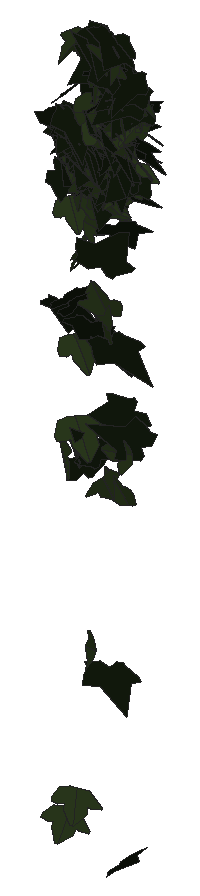
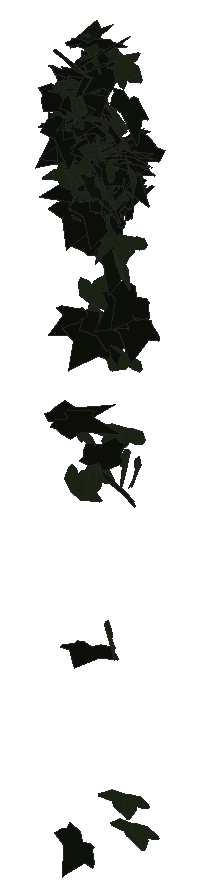
# SketchUp Ruby script. Lengths in inches.
U = 1.inch
M = Sketchup.active_model
def pt(a) = Geom::Point3d.new(a.map { |v| v * U })
def face(e, loops, mat)
  f = e.add_face(loops[0].map { |a| pt(a) })
  loops[1..].each { |l| e.add_face(l.map { |a| pt(a) }).erase! }
  f.material = f.back_material = mat if mat
  f
end
# faces: each face lists its corners as indices into pts; further lists are holes
def faces(e, pts, list, mat = nil) = list.each { |f| face(e, (f[0].is_a?(Array) ? f : [f]).map { |l| l.map { |i| pts[i] } }, mat) }
# xy, xz, yz: faces in a plane at the given z, y or x. An outline is a flat list of corners, or four numbers for a rectangle; further outlines are holes
def ring(l) = l.size == 4 ? [[l[0], l[1]], [l[2], l[1]], [l[2], l[3]], [l[0], l[3]]] : l.each_slice(2).to_a
def flat(e, list, mat, &to3) = list.each { |f| face(e, (f[0].is_a?(Array) ? f : [f]).map { |l| ring(l).map { |u, v| to3.(u, v) } }, mat) }
def xy(e, z, list, mat = nil) = flat(e, list, mat) { |x, y| [x, y, z] }
def xz(e, y, list, mat = nil) = flat(e, list, mat) { |x, z| [x, y, z] }
def yz(e, x, list, mat = nil) = flat(e, list, mat) { |y, z| [x, y, z] }
def lines(e, pts, list) = list.each { |a, b| e.add_line(pt(pts[a]), pt(pts[b])) }
# prism: a flat outline (further loops are holes) pulled along v
def prism(e, loops, v, mat = nil)
  f = face(e, loops, mat); d = Geom::Vector3d.new(v.map { |x| x * U })
  f.pushpull(f.normal.samedirection?(d) ? d.length : -d.length)
end
def box(e, o, s, mat = nil) = prism(e, [[o, [o[0] + s[0], o[1], o[2]], [o[0] + s[0], o[1] + s[1], o[2]], [o[0], o[1] + s[1], o[2]]]], [0, 0, s[2]], mat)
def at(x, y, z, deg = 0) = Geom::Transformation.translation(pt([x, y, z])) * Geom::Transformation.rotation(ORIGIN, Z_AXIS, deg.degrees)
def axes(o, x, y, z) = Geom::Transformation.new([*x, 0, *y, 0, *z, 0, *pt(o).to_a, 1])
def part(name) = M.definitions.add(name)
# library, detail: a bought-in or finely detailed component or shape, given as its bounding box
def library(name, o, s) = part(name).tap { |d| box(d.entities, o, s) }
def detail(e, o, s) = box(e.add_group.entities, o, s)
def put(e, d, t, mat = nil) = e.add_instance(d, t).tap { |i| i.material = mat if mat }
def group(e, t, mat = nil) = e.add_group.tap { |g| g.transformation = t; g.material = mat if mat }.entities
root = M.entities
M.materials.add("1026 AP 7946 SUNNY SIDE UP").color = [254, 231, 186]
M.materials.add("efeu1").color = [18, 25, 13]
M.materials.add("efeu2").color = [43, 57, 29]
c1 = part("ivyleaf_9")
p = [[1.54,2.16,1.25],[1.36,2.04,1.19],[-0.21,0.99,0.68],[-0.71,1.11,0.82],[-0.85,0.86,0.67],[-0.8,0.17,0.21],
  [-0.9,-0.01,0.1],[-0.67,-0.16,-0.02],[-0.08,-0.08,-0.05],[-0.03,-0.6,-0.4],[0.65,-0.88,-0.66],[0.83,-0.6,-0.49],
  [1.29,-0.42,-0.43],[1.8125,-0.07,-0.26],[1.21,0.44,0.15]]
faces(c1.entities,p,[[0,1,2,3,4,5,6,7,8,9,10,11,12,13,14]],"efeu1")
c2 = part("ivyleaf_10")
p = [[0,0.5,-0.03],[-0.0625,2.02,-0.43],[-0.19,2.01,-0.46],[-0.54,1.05,-0.29],[-0.52,0.625,-0.18],[-0.83,0.76,-0.28],
  [-1.16,0.64,-0.33],[-1.15,0.33,-0.24],[-0.77,-0.39,0.02],[-0.3,-0.51,0.16],[0.04,-0.48,0.23],[-0.02,2.01,-0.4375],
  [-0.06,2.01,-0.43],[0.04,-0.49,0.23],[0.67,-0.49,0.14],[1.38,0.36,-0.2],[1.375,0.51,-0.24],[0.81,0.65,-0.19],
  [0.62,0.59,-0.15],[0.6,1.09,-0.28],[0.5,1.23,-0.31]]
faces(c2.entities,p,[[0,1,2,3,4,5,6,7,8,9,10],[11,12,0,13,14,15,16,17,18,19,20]],"efeu2")
put(root,c1,axes([114.61,212.93,265.6875],[-0.05333,0.19687,-0.14249],[-0.05578,-0.14334,-0.20046],[-0.37521,-0.00667,0.05006]),"1026 AP 7946 SUNNY SIDE UP")
put(root,c2,axes([114.4,212.68,259.63],[-0.11326,0.21899,-0.07805],[0.0251,-0.07577,-0.23779],[-0.36414,-0.07333,0.00789]),"1026 AP 7946 SUNNY SIDE UP")
put(root,c1,axes([114.48,212.61,262.48],[0.29734,0.09526,-0.11901],[-0.13937,-0.07983,-0.21675],[-0.19058,0.20702,-0.02717]),"1026 AP 7946 SUNNY SIDE UP")
put(root,c2,axes([114.38,212.92,264.26],[0.24145,0.1835,0.03806],[0.03802,0.02658,-0.24634],[-0.29154,0.15544,-0.00061]),"1026 AP 7946 SUNNY SIDE UP")
put(root,c1,axes([114.33,212.96,265.49],[0.20834,-0.19966,-0.05353],[-0.06361,0.03404,-0.2462],[0.31765,0.13777,-0.01419]),"1026 AP 7946 SUNNY SIDE UP")
put(root,c1,axes([114.4,212.9,264.9375],[-0.05589,-0.1113,0.21897],[-0.01073,-0.21494,-0.11804],[0.37799,-0.02256,0.02903]),"1026 AP 7946 SUNNY SIDE UP")
put(root,c2,axes([114.48,212.67,252.5],[0.38235,0.02143,-0.02276],[-0.03132,-0.02579,-0.25042],[-0.03706,0.24281,-0.02314]),"1026 AP 7946 SUNNY SIDE UP")
put(root,c2,axes([114.51,212.85,265.91],[0.15682,-0.22679,-0.00735],[0.02996,0.01473,-0.25401],[0.35547,0.09881,0.02465]),"1026 AP 7946 SUNNY SIDE UP")
put(root,c1,axes([114.4,212.53,265.07],[0.19369,-0.10602,-0.21035],[-0.11166,0.20211,-0.15151],[0.34322,0.12558,0.06942]),"1026 AP 7946 SUNNY SIDE UP")
put(root,c2,axes([114.41,212.9,265.57],[-0.23643,0.11477,-0.15666],[0.1408,-0.12933,-0.19171],[-0.26535,-0.17089,0.03785]),"1026 AP 7946 SUNNY SIDE UP")
put(root,c1,axes([114.32,212.95,265.11],[0.05251,-0.03831,-0.24539],[0.35496,-0.07926,0.04532],[-0.13288,-0.22686,0.02408]),"1026 AP 7946 SUNNY SIDE UP")
put(root,c1,axes([114.56,212.96,265.89],[-0.22943,-0.19387,0.04254],[-0.02691,-0.04013,-0.24998],[0.31089,-0.14655,0.00976]),"1026 AP 7946 SUNNY SIDE UP")
put(root,c1,axes([114.67,212.5625,266.77],[-0.03368,0.24703,0.04677],[-0.00032,0.04414,-0.25516],[-0.39454,-0.02112,-0.00379]),"1026 AP 7946 SUNNY SIDE UP")
put(root,c1,axes([114.38,212.9375,265.44],[0.05893,-0.23241,0.06215],[0.02788,-0.05956,-0.24274],[0.37706,0.04073,0.00823]),"1026 AP 7946 SUNNY SIDE UP")
put(root,c1,axes([114.52,212.97,265.73],[-0.26587,-0.16572,-0.06851],[0.10124,0.02747,-0.24243],[0.26131,-0.17926,0.02422]),"1026 AP 7946 SUNNY SIDE UP")
put(root,c1,axes([114.57,212.93,266],[-0.32539,-0.13596,-0.02618],[0.09505,-0.04918,-0.24373],[0.19538,-0.20251,0.07498]),"1026 AP 7946 SUNNY SIDE UP")
put(root,c2,axes([114.57,212.86,267.61],[-0.01298,-0.17717,0.19164],[0.02965,-0.18704,-0.18277],[0.404,0.00804,0.01957]),"1026 AP 7946 SUNNY SIDE UP")
put(root,c2,axes([114.62,212.98,265.69],[-0.04034,-0.24068,0.0225],[-0.00023,-0.02332,-0.24948],[0.38021,-0.02555,0.00224]),"1026 AP 7946 SUNNY SIDE UP")
put(root,c2,axes([114.63,212.68,259.76],[-0.18763,0.19887,0.07935],[-0.0833,0.05653,-0.23806],[-0.32418,-0.12963,0.01524]),"1026 AP 7946 SUNNY SIDE UP")
put(root,c1,axes([114.26,212.67,265.8125],[0.08907,0.00515,0.27764],[0.41543,-0.05551,-0.05645],[0.0838,0.26971,-0.01527]),"1026 AP 7946 SUNNY SIDE UP")
put(root,c1,axes([114.58,212.9375,265.39],[0.2485,-0.09589,-0.16561],[-0.232,0.0645,-0.18933],[0.17992,0.2156,-0.01539]),"1026 AP 7946 SUNNY SIDE UP")
put(root,c2,axes([114.57,212.83,265.39],[-0.13838,0.1416,-0.1832],[0.06251,-0.17902,-0.16742],[-0.35294,-0.08723,0.04218]),"1026 AP 7946 SUNNY SIDE UP")
put(root,c1,axes([114.65,212.93,265.84],[-0.29389,-0.15418,-0.05522],[0.11125,-0.00451,-0.24481],[0.23081,-0.19415,0.04769]),"1026 AP 7946 SUNNY SIDE UP")
put(root,c1,axes([114.76,212.8,259.25],[-0.30001,0.16468,-0.05193],[-0.04194,0.04746,0.25926],[0.26798,0.1918,-0.01756]),"1026 AP 7946 SUNNY SIDE UP")
put(root,c2,axes([114.68,212.7,265.36],[0.34307,-0.10812,0.00827],[0.0109,-0.00548,-0.25088],[0.17021,0.21828,-0.00061]),"1026 AP 7946 SUNNY SIDE UP")
put(root,c1,axes([114.93,212.875,266.33],[-0.01864,0.08351,0.28829],[-0.1234,0.26837,-0.0845],[-0.44157,-0.07852,0.01144]),"1026 AP 7946 SUNNY SIDE UP")
put(root,c2,axes([114.74,212.74,263.66],[0.11866,-0.23815,0.02219],[-0.00014,-0.02403,-0.2574],[0.3762,0.07511,-0.00709]),"1026 AP 7946 SUNNY SIDE UP")
put(root,c1,axes([114.6875,212.38,262.79],[0.15853,0.20494,0.11603],[0.08576,0.09736,-0.23466],[-0.35667,0.1145,-0.00485]),"1026 AP 7946 SUNNY SIDE UP")
put(root,c1,axes([114.64,212.81,265.91],[-0.03721,-0.25365,0.0092],[-0.00123,-0.01034,-0.2625],[0.39917,-0.02367,0.00005]),"1026 AP 7946 SUNNY SIDE UP")
put(root,c1,axes([114.63,212.73,266.125],[-0.03918,-0.25802,-0.01343],[0.01169,0.01091,-0.2669],[0.40595,-0.02522,0.00639]),"1026 AP 7946 SUNNY SIDE UP")
put(root,c1,axes([114.51,212.75,265.2],[0.08159,-0.14421,0.1985],[0.18514,-0.15764,-0.15448],[0.33125,0.12363,0.03745]),"1026 AP 7946 SUNNY SIDE UP")
put(root,c2,axes([114.7,212.63,252.99],[0.3606,0.08865,0.00222],[0.01499,-0.0201,-0.25238],[-0.13862,0.22845,-0.02152]),"1026 AP 7946 SUNNY SIDE UP")
put(root,c2,axes([114.89,212.9,264.64],[-0.13289,0.18179,-0.14206],[-0.07009,0.13219,0.20689],[0.35287,0.09472,-0.0124]),"1026 AP 7946 SUNNY SIDE UP")
put(root,c2,axes([114.78,212.74,264.92],[0.0278,-0.23922,0.07096],[0.08375,-0.06516,-0.24284],[0.38298,0.03161,0.04795]),"1026 AP 7946 SUNNY SIDE UP")
put(root,c2,axes([114.85,212.97,265.15],[-0.26828,-0.16192,0.05873],[0.01197,-0.08862,-0.23265],[0.27014,-0.15688,0.06863]),"1026 AP 7946 SUNNY SIDE UP")
put(root,c1,axes([114.48,212.72,265.46],[0.18973,-0.0468,0.21691],[0.3205,-0.05508,-0.13311],[0.11215,0.23658,0.01344]),"1026 AP 7946 SUNNY SIDE UP")
put(root,c1,axes([114.73,212.49,262.6],[0.17535,0.16565,0.16747],[0.15173,0.12979,-0.20487],[-0.33077,0.14735,-0.0052]),"1026 AP 7946 SUNNY SIDE UP")
put(root,c2,axes([114.83,212.8125,266.27],[-0.3042,0.1507,-0.04565],[0.01363,-0.06128,-0.24921],[-0.247,-0.18898,0.04247]),"1026 AP 7946 SUNNY SIDE UP")
put(root,c1,axes([114.96,212.83,264.88],[-0.05574,0.23506,-0.05008],[0.01517,-0.04906,-0.24517],[-0.37755,-0.03668,-0.00246]),"1026 AP 7946 SUNNY SIDE UP")
put(root,c2,axes([114.87,212.81,264.09],[-0.03218,0.1479,0.19779],[-0.07189,0.186,-0.15222],[-0.37317,-0.04859,0.01227]),"1026 AP 7946 SUNNY SIDE UP")
put(root,c2,axes([114.89,212.9,265.23],[-0.38207,0.01484,-0.00804],[0.00996,-0.02498,-0.24966],[-0.02447,-0.24183,0.02386]),"1026 AP 7946 SUNNY SIDE UP")
put(root,c1,axes([114.6875,212.79,266.02],[0.09518,-0.22147,-0.1124],[0.01517,0.1131,-0.23304],[0.38704,0.05003,0.03678]),"1026 AP 7946 SUNNY SIDE UP")
put(root,c2,axes([114.875,213.02,265.18],[0.2676,-0.17225,-0.00356],[-0.02,-0.00909,-0.249],[0.27014,0.16996,-0.0149]),"1026 AP 7946 SUNNY SIDE UP")
put(root,c2,axes([114.68,212.6875,261.77],[0.33154,0.05044,0.11661],[0.18183,-0.00137,-0.22185],[-0.06887,0.23917,-0.0244]),"1026 AP 7946 SUNNY SIDE UP")
put(root,c1,axes([114.71,212.96,265.08],[0.28332,-0.1529,-0.05402],[-0.08159,0.01829,-0.24254],[0.24026,0.18652,-0.01866]),"1026 AP 7946 SUNNY SIDE UP")
put(root,c2,axes([114.85,212.8125,265.87],[-0.2475,0.16871,-0.08167],[0.02355,-0.09318,-0.23267],[-0.29281,-0.1501,0.05032]),"1026 AP 7946 SUNNY SIDE UP")
put(root,c1,axes([114.95,212.61,263.55],[0.03202,0.21052,0.12117],[0.0253,0.11539,-0.21717],[-0.37743,0.0256,-0.00428]),"1026 AP 7946 SUNNY SIDE UP")
put(root,c2,axes([114.97,212.95,265.19],[-0.14866,0.19543,-0.11407],[-0.06012,0.1056,0.22402],[0.34891,0.10146,-0.01]),"1026 AP 7946 SUNNY SIDE UP")
put(root,c1,axes([114.93,212.94,265.96],[0.23203,0.1536,-0.13166],[-0.12227,-0.10339,-0.21961],[-0.29038,0.16627,-0.01274]),"1026 AP 7946 SUNNY SIDE UP")
put(root,c1,axes([115.07,213.09,265.3],[-0.20652,0.19986,-0.04085],[0.01727,-0.04151,-0.24623],[-0.32027,-0.13111,0.01306]),"1026 AP 7946 SUNNY SIDE UP")
put(root,c2,axes([114.93,212.94,266.05],[0.02504,-0.24775,0.0172],[0.00001,-0.01814,-0.25586],[0.3906,0.01588,-0.0011]),"1026 AP 7946 SUNNY SIDE UP")
put(root,c2,axes([114.76,212.62,260.21],[0.334,0.18375,0.07203],[0.10084,0.03092,-0.28857],[-0.29161,0.22115,-0.01729]),"1026 AP 7946 SUNNY SIDE UP")
put(root,c1,axes([114.87,212.87,265.4],[-0.18611,-0.19906,0.08068],[0.03078,-0.10042,-0.22974],[0.3356,-0.10118,0.06581]),"1026 AP 7946 SUNNY SIDE UP")
put(root,c2,axes([114.89,212.96,265.98],[0.10266,0.23432,0.02189],[-0.04252,0.02802,-0.24804],[-0.36732,0.06225,0.03483]),"1026 AP 7946 SUNNY SIDE UP")
put(root,c2,axes([115.02,212.8,266.08],[-0.38502,-0.02737,0.04223],[-0.05837,-0.03546,-0.25206],[0.0513,-0.24575,0.03018]),"1026 AP 7946 SUNNY SIDE UP")
put(root,c1,axes([114.96,212.93,264.72],[0.21896,0.19792,-0.02089],[-0.02267,-0.01603,-0.24938],[-0.3122,0.13997,0.00345]),"1026 AP 7946 SUNNY SIDE UP")
put(root,c1,axes([115.08,212.84,259.62],[0.08433,0.07602,0.2382],[-0.33777,-0.09562,0.08332],[0.17857,-0.21678,0.04511]),"1026 AP 7946 SUNNY SIDE UP")
put(root,c1,axes([115.05,212.62,262.3],[0.23705,0.12612,-0.15074],[-0.16469,-0.10366,-0.20284],[-0.25624,0.18331,-0.00908]),"1026 AP 7946 SUNNY SIDE UP")
put(root,c2,axes([114.85,213,265.86],[-0.25529,-0.0927,-0.16368],[0.24332,0.04445,-0.19],[0.15505,-0.22239,0.02867]),"1026 AP 7946 SUNNY SIDE UP")
put(root,c2,axes([115.11,212.96,266.29],[0.32827,0.02276,0.13846],[-0.21258,0.06432,0.20569],[-0.02587,-0.23975,0.06682]),"1026 AP 7946 SUNNY SIDE UP")
put(root,c2,axes([115.07,212.93,264.84],[-0.29961,-0.14912,0.02503],[-0.00703,-0.03487,-0.24818],[0.23768,-0.18901,0.02421]),"1026 AP 7946 SUNNY SIDE UP")
put(root,c2,axes([115.17,212.5,256.06],[0.06665,-0.12895,-0.21331],[-0.12497,0.19061,-0.13842],[0.36159,0.08965,-0.00852]),"1026 AP 7946 SUNNY SIDE UP")
put(root,c1,axes([114.76,212.86,265.2],[0.24522,-0.13562,0.1399],[0.16156,-0.08997,-0.21344],[0.25591,0.18676,0.00069]),"1026 AP 7946 SUNNY SIDE UP")
put(root,c1,axes([115.01,212.94,265.19],[-0.1568,-0.22076,-0.03475],[0.03041,0.02689,-0.2493],[0.34954,-0.10137,0.0061]),"1026 AP 7946 SUNNY SIDE UP")
put(root,c1,axes([114.93,212.82,265.54],[-0.1144,-0.20793,-0.10875],[0.11692,0.08285,-0.22293],[0.34665,-0.09656,0.0393]),"1026 AP 7946 SUNNY SIDE UP")
put(root,c1,axes([114.92,212.89,267.48],[0.38577,-0.06396,-0.05691],[-0.0895,-0.00116,-0.26073],[0.09773,0.2514,-0.01412]),"1026 AP 7946 SUNNY SIDE UP")
put(root,c1,axes([114.99,212.875,265.6875],[-0.12643,-0.22771,0.02802],[0.05707,-0.04243,-0.24406],[0.3563,-0.074,0.04904]),"1026 AP 7946 SUNNY SIDE UP")
put(root,c2,axes([114.83,212.67,266.32],[0.16208,-0.09875,-0.23884],[0.30099,-0.13131,0.14488],[-0.25646,-0.21651,0.01908]),"1026 AP 7946 SUNNY SIDE UP")
put(root,c1,axes([115.2,212.8125,267.34],[-0.24379,-0.14274,0.14803],[-0.10433,-0.13622,-0.21277],[0.30186,-0.16236,0.04601]),"1026 AP 7946 SUNNY SIDE UP")
put(root,c1,axes([114.96,212.98,265.28],[0.07686,-0.23614,0.02947],[0.0052,-0.0299,-0.24858],[0.37424,0.04891,-0.0026]),"1026 AP 7946 SUNNY SIDE UP")
put(root,c1,axes([115.28,212.94,266.57],[0.07369,-0.06612,0.24353],[-0.14213,0.21951,0.08287],[-0.35945,-0.10035,0.01716]),"1026 AP 7946 SUNNY SIDE UP")
put(root,c1,axes([115.41,212.93,265.37],[-0.31181,0.03871,0.14284],[-0.22573,-0.04133,-0.20019],[-0.01151,-0.23829,0.05645]),"1026 AP 7946 SUNNY SIDE UP")
put(root,c1,axes([115.13,212.76,264.99],[0.27223,0.16036,-0.08055],[-0.07012,-0.0679,-0.24276],[-0.27228,0.17782,-0.01802]),"1026 AP 7946 SUNNY SIDE UP")
put(root,c1,axes([115.02,212.89,265.58],[-0.01313,-0.22406,0.11141],[-0.00308,-0.10942,-0.23162],[0.39207,-0.00836,0.00191]),"1026 AP 7946 SUNNY SIDE UP")
put(root,c2,axes([115.16,212.76,267.15],[0.04538,0.24872,-0.06666],[-0.08759,-0.05892,-0.25372],[-0.39508,0.04163,0.04859]),"1026 AP 7946 SUNNY SIDE UP")
put(root,c1,axes([114.93,212.9,265.65],[0.33593,-0.11466,0.02753],[0.02231,-0.03125,-0.24905],[0.18401,0.21311,-0.02007]),"1026 AP 7946 SUNNY SIDE UP")
put(root,c2,axes([115.1,212.58,267.62],[-0.36933,0.08549,-0.0903],[0.11198,-0.06013,-0.25596],[-0.15728,-0.24356,0.02981]),"1026 AP 7946 SUNNY SIDE UP")
put(root,c2,axes([115.22,212.8125,267.37],[-0.38812,0.06465,0.01672],[-0.03349,-0.01897,-0.26184],[-0.09916,-0.24662,0.02297]),"1026 AP 7946 SUNNY SIDE UP")
put(root,c2,axes([115.16,212.99,265.55],[0.1832,0.20687,-0.05781],[-0.03268,-0.05401,-0.24476],[-0.33593,0.11807,-0.00772]),"1026 AP 7946 SUNNY SIDE UP")
put(root,c2,axes([115.33,212.64,262.68],[-0.35797,-0.04473,-0.08571],[-0.13516,0.00968,0.23773],[-0.06073,0.24211,-0.02388]),"1026 AP 7946 SUNNY SIDE UP")
put(root,c1,axes([115.03,212.83,266.2],[0.14808,-0.2279,-0.03514],[-0.01005,0.03285,-0.25375],[0.36191,0.09416,0.00733]),"1026 AP 7946 SUNNY SIDE UP")
put(root,c2,axes([115.27,212.77,265.125],[-0.05594,-0.24108,0.06399],[-0.01806,-0.06247,-0.2514],[0.39158,-0.03732,-0.00245]),"1026 AP 7946 SUNNY SIDE UP")
put(root,c1,axes([115.15,212.79,266.94],[0.33278,-0.05017,-0.14409],[-0.19931,0.06511,-0.22173],[0.1211,0.24502,0.03102]),"1026 AP 7946 SUNNY SIDE UP")
put(root,c1,axes([114.97,212.93,266.1875],[0.2722,-0.18046,0.01183],[0.04273,0.00882,-0.25621],[0.28122,0.17334,0.02748]),"1026 AP 7946 SUNNY SIDE UP")
put(root,c1,axes([115.17,212.91,264.82],[-0.13568,-0.2269,0.02564],[-0.00414,-0.02699,-0.25013],[0.35912,-0.08604,0.0068]),"1026 AP 7946 SUNNY SIDE UP")
put(root,c1,axes([115.27,212.5625,267.3],[0.13733,0.23536,-0.04172],[-0.0031,-0.04383,-0.25852],[-0.37587,0.08636,-0.01311]),"1026 AP 7946 SUNNY SIDE UP")
put(root,c1,axes([115.1,212.85,265.53],[0.20562,-0.20374,-0.02976],[-0.0474,0.01352,-0.24864],[0.31982,0.13299,-0.01772]),"1026 AP 7946 SUNNY SIDE UP")
put(root,c1,axes([115.46,213.22,260.48],[-0.0242,-0.06324,-0.24769],[-0.11935,-0.22781,0.0655],[-0.37167,0.07727,-0.00491]),"1026 AP 7946 SUNNY SIDE UP")
put(root,c2,axes([115,212.71,264.65],[-0.10855,-0.03925,-0.24214],[0.37434,-0.00918,-0.07057],[0.00337,-0.24459,0.04004]),"1026 AP 7946 SUNNY SIDE UP")
put(root,c1,axes([115.15,213,266.06],[0.07221,-0.24151,-0.00828],[-0.00064,0.00671,-0.25322],[0.3799,0.04592,0.00115]),"1026 AP 7946 SUNNY SIDE UP")
put(root,c2,axes([115.28,212.69,259.29],[-0.10549,-0.2152,-0.11299],[0.08576,0.09611,-0.23063],[0.36909,-0.08384,0.02129]),"1026 AP 7946 SUNNY SIDE UP")
put(root,c1,axes([115.48,212.71,267.3],[-0.14567,-0.27237,0.01793],[0.01225,0.01737,0.29648],[-0.42914,0.09295,0.00237]),"1026 AP 7946 SUNNY SIDE UP")
put(root,c2,axes([115.54,212.49,262.43],[-0.02043,0.03666,0.27922],[-0.36103,0.1456,-0.0308],[-0.2331,-0.22873,0.02323]),"1026 AP 7946 SUNNY SIDE UP")
put(root,c1,axes([115.48,212.66,265.69],[-0.27079,0.18275,-0.06541],[0.04994,-0.05854,-0.25847],[-0.30062,-0.17434,0.01598]),"1026 AP 7946 SUNNY SIDE UP")
put(root,c1,axes([115.3,212.85,267.86],[-0.26157,-0.19792,-0.02767],[0.07645,-0.00769,-0.26286],[0.30438,-0.16815,0.04225]),"1026 AP 7946 SUNNY SIDE UP")
put(root,c1,axes([115.38,212.76,266.62],[0.13024,0.23088,-0.05608],[-0.01378,-0.05603,-0.2528],[-0.37322,0.08264,-0.01024]),"1026 AP 7946 SUNNY SIDE UP")
put(root,c1,axes([115.17,212.875,266.49],[0.3977,0.02099,-0.00689],[-0.00901,-0.01318,-0.26121],[-0.0335,0.25267,-0.01156]),"1026 AP 7946 SUNNY SIDE UP")
put(root,c2,axes([115.55,212.88,258.97],[-0.327,0.06018,-0.12649],[-0.17748,0.0517,0.22273],[0.12222,0.23608,-0.01499]),"1026 AP 7946 SUNNY SIDE UP")
put(root,c2,axes([115.54,212.62,267.6],[0.15035,-0.12775,-0.24067],[-0.19854,0.19591,-0.16297],[0.36747,0.15811,0.01042]),"1026 AP 7946 SUNNY SIDE UP")
put(root,c2,axes([115.42,212.82,265.34],[-0.18996,-0.21873,-0.03148],[0.04097,0.01906,-0.25693],[0.34457,-0.12285,0.01319]),"1026 AP 7946 SUNNY SIDE UP")
put(root,c2,axes([115.41,212.9,265.02],[0.05053,0.15617,-0.19197],[-0.07944,-0.18049,-0.16507],[-0.37504,0.05927,0.0091]),"1026 AP 7946 SUNNY SIDE UP")
put(root,c1,axes([115.31,212.88,266],[-0.01733,-0.24281,0.04933],[-0.00572,-0.04914,-0.25068],[0.38953,-0.01153,-0.00149]),"1026 AP 7946 SUNNY SIDE UP")
put(root,c1,axes([115.32,212.71,261.94],[0.37397,0.03451,-0.05884],[-0.08484,-0.02622,-0.24706],[-0.0622,0.24323,-0.01681]),"1026 AP 7946 SUNNY SIDE UP")
put(root,c2,axes([115.47,212.9,265.07],[-0.04125,-0.24482,0.00471],[0.00297,-0.0062,-0.25368],[0.38506,-0.02618,0.00246]),"1026 AP 7946 SUNNY SIDE UP")
put(root,c2,axes([115.3125,212.6875,264.8],[-0.30387,-0.0746,-0.14296],[0.21683,0.02473,-0.21204],[0.11858,-0.23638,0.0214]),"1026 AP 7946 SUNNY SIDE UP")
put(root,c2,axes([115.24,212.66,266.18],[0.31408,0.14115,0.14144],[0.18437,0.07042,-0.25139],[-0.24765,0.23145,-0.00778]),"1026 AP 7946 SUNNY SIDE UP")
put(root,c1,axes([115.36,212.53,263.6],[-0.26,0.01378,0.21261],[0.32375,-0.01314,0.17084],[0.02967,0.26406,-0.00104]),"1026 AP 7946 SUNNY SIDE UP")
put(root,c2,axes([115.48,212.88,265.84],[0.36713,-0.06143,-0.03996],[-0.06419,-0.00436,-0.2483],[0.09414,0.23659,-0.01348]),"1026 AP 7946 SUNNY SIDE UP")
put(root,c2,axes([115.41,212.82,266.35],[0.37806,0.05306,0.01612],[0.01626,0.0241,-0.25257],[-0.08531,0.23972,0.02331]),"1026 AP 7946 SUNNY SIDE UP")
put(root,c1,axes([115.24,212.86,264.96],[0.3205,0.04653,0.13242],[0.20759,-0.00897,-0.21282],[-0.05422,0.24066,-0.03207]),"1026 AP 7946 SUNNY SIDE UP")
put(root,c2,axes([115.56,212.9,266.33],[-0.07281,-0.24778,-0.00358],[0.00376,0.00166,-0.25966],[0.3896,-0.04632,0.00183]),"1026 AP 7946 SUNNY SIDE UP")
put(root,c1,axes([115.29,212.82,265.75],[0.32661,0.06325,0.12843],[0.18302,0.04423,-0.2233],[-0.12081,0.23799,0.00891]),"1026 AP 7946 SUNNY SIDE UP")
put(root,c1,axes([115.46,212.79,267.81],[-0.15283,-0.18458,0.17047],[0.04089,-0.18537,-0.19712],[0.38875,-0.05307,0.08775]),"1026 AP 7946 SUNNY SIDE UP")
put(root,c2,axes([115.66,212.93,266.55],[-0.26216,0.14723,0.12283],[-0.17053,0.05472,-0.22711],[-0.24326,-0.19703,0.02683]),"1026 AP 7946 SUNNY SIDE UP")
put(root,c2,axes([115.74,212.65,260.01],[0.13674,-0.09541,-0.22012],[-0.25673,0.13774,-0.13135],[0.26248,0.18442,-0.0138]),"1026 AP 7946 SUNNY SIDE UP")
put(root,c2,axes([115.48,212.81,266.74],[0.12178,-0.21785,0.10209],[0.10193,-0.0825,-0.23656],[0.3631,0.09623,0.03217]),"1026 AP 7946 SUNNY SIDE UP")
put(root,c2,axes([115.625,212.89,265.18],[-0.36186,0.08822,0.01519],[-0.08431,-0.10485,-0.22414],[-0.11241,-0.20536,0.11923]),"1026 AP 7946 SUNNY SIDE UP")
put(root,c2,axes([115.53,212.98,266.4375],[0.2419,-0.18422,-0.05901],[0.01162,0.07757,-0.24048],[0.30263,0.14427,0.05641]),"1026 AP 7946 SUNNY SIDE UP")
put(root,c1,axes([115.55,212.8,251.87],[0.10591,0.21464,0.13525],[0.07734,0.12077,-0.23085],[-0.38698,0.08288,-0.00912]),"1026 AP 7946 SUNNY SIDE UP")
put(root,c1,axes([115.64,212.86,265.3],[-0.36571,-0.00458,-0.08013],[0.11969,-0.06523,-0.231],[-0.02595,-0.2364,0.0638]),"1026 AP 7946 SUNNY SIDE UP")
put(root,c1,axes([115.45,212.99,266.35],[-0.0122,-0.24652,-0.0234],[-0.00126,0.02135,-0.25396],[0.38908,-0.00766,-0.00155]),"1026 AP 7946 SUNNY SIDE UP")
put(root,c1,axes([115.3125,212.9375,266.4],[0.35068,-0.11056,0.03346],[0.07938,0.02867,-0.25152],[0.1632,0.22364,0.05044]),"1026 AP 7946 SUNNY SIDE UP")
put(root,c1,axes([115.47,212.625,255.7],[-0.13874,-0.18419,-0.149],[0.13137,0.11844,-0.20872],[0.34292,-0.11989,0.01967]),"1026 AP 7946 SUNNY SIDE UP")
put(root,c1,axes([115.57,212.69,264.34],[0.26689,0.17336,-0.02561],[-0.0095,-0.03018,-0.24952],[-0.27543,0.16902,-0.01622]),"1026 AP 7946 SUNNY SIDE UP")
put(root,c2,axes([115.59,213.12,265.28],[0.27694,0.1554,-0.06557],[-0.05412,-0.05817,-0.24142],[-0.25898,0.17833,-0.01967]),"1026 AP 7946 SUNNY SIDE UP")
put(root,c1,axes([115.69,212.99,266.11],[0.08111,0.24078,-0.01568],[0.00366,-0.01746,-0.25371],[-0.37948,0.0513,-0.0058]),"1026 AP 7946 SUNNY SIDE UP")
put(root,c1,axes([115.43,212.76,265.92],[0.13153,-0.2254,0.07218],[0.03889,-0.06691,-0.24807],[0.36971,0.08723,0.00042]),"1026 AP 7946 SUNNY SIDE UP")
put(root,c1,axes([115.77,212.77,266.91],[-0.38257,-0.06599,0.0047],[0.00234,-0.02426,-0.25868],[0.10402,-0.24214,0.0231]),"1026 AP 7946 SUNNY SIDE UP")
put(root,c2,axes([115.74,212.64,266.28],[-0.00838,0.02532,-0.26908],[-0.07206,0.25729,0.02815],[0.40652,0.04613,-0.00055]),"1026 AP 7946 SUNNY SIDE UP")
put(root,c1,axes([115.82,212.87,267.1],[-0.392,-0.04067,0.01358],[-0.01551,-0.02257,-0.25948],[0.06553,-0.24864,0.01983]),"1026 AP 7946 SUNNY SIDE UP")
put(root,c2,axes([115.73,212.98,266.7],[-0.3845,0.0499,0.02286],[-0.05273,-0.0584,-0.24894],[-0.06755,-0.23846,0.06421]),"1026 AP 7946 SUNNY SIDE UP")
put(root,c1,axes([115.55,212.78,265.43],[-0.24022,-0.06622,-0.19321],[0.30599,-0.00312,-0.16251],[0.06189,-0.24158,0.05354]),"1026 AP 7946 SUNNY SIDE UP")
put(root,c2,axes([115.71,212.83,265.8125],[0.00127,-0.22619,0.10445],[-0.00049,-0.10268,-0.23362],[0.39059,0.00061,-0.00063]),"1026 AP 7946 SUNNY SIDE UP")
put(root,c1,axes([115.92,212.83,260.13],[-0.07275,0.01946,0.26537],[-0.38126,-0.09324,-0.03817],[0.13965,-0.24443,0.03405]),"1026 AP 7946 SUNNY SIDE UP")
put(root,c1,axes([115.51,212.98,265.9],[0.42424,0.02587,0.00301],[0.00826,-0.02585,-0.27807],[-0.04008,0.26858,-0.02545]),"1026 AP 7946 SUNNY SIDE UP")
put(root,c1,axes([115.87,212.92,266.7],[-0.00251,0.20873,-0.13826],[-0.05451,-0.13426,-0.2136],[-0.38739,0.01754,0.03095]),"1026 AP 7946 SUNNY SIDE UP")
put(root,c2,axes([115.6875,212.94,266.76],[-0.2897,0.16211,-0.05899],[0.04432,-0.05567,-0.25207],[-0.26717,-0.18501,0.02215]),"1026 AP 7946 SUNNY SIDE UP")
put(root,c1,axes([115.76,212.92,266.73],[-0.27484,-0.18131,0.01315],[0.00516,-0.02227,-0.25893],[0.28587,-0.17391,0.01732]),"1026 AP 7946 SUNNY SIDE UP")
put(root,c1,axes([115.51,212.77,266.02],[0.3202,-0.13966,0.012],[0.00018,-0.02178,-0.25384],[0.22047,0.20285,-0.01722]),"1026 AP 7946 SUNNY SIDE UP")
put(root,c1,axes([115.78,212.89,265.3],[-0.29505,-0.1459,0.07074],[0.01853,-0.11856,-0.22435],[0.25344,-0.16119,0.09875]),"1026 AP 7946 SUNNY SIDE UP")
put(root,c1,axes([115.77,212.83,267.29],[-0.34418,-0.03521,-0.14222],[0.22367,-0.04852,-0.22019],[0.00499,-0.25409,0.06019]),"1026 AP 7946 SUNNY SIDE UP")
put(root,c2,axes([115.64,212.75,266.76],[-0.23706,-0.13664,-0.15488],[0.22806,0.05736,-0.20427],[0.22239,-0.20447,0.04438]),"1026 AP 7946 SUNNY SIDE UP")
put(root,c1,axes([115.56,212.57,262.13],[-0.07898,-0.08518,-0.25339],[0.2695,0.17706,-0.09839],[0.30709,-0.17729,0.02117]),"1026 AP 7946 SUNNY SIDE UP")
put(root,c2,axes([115.83,212.95,266.35],[-0.13776,-0.12605,0.20238],[0.02748,-0.21347,-0.13384],[0.36694,-0.03134,0.086]),"1026 AP 7946 SUNNY SIDE UP")
